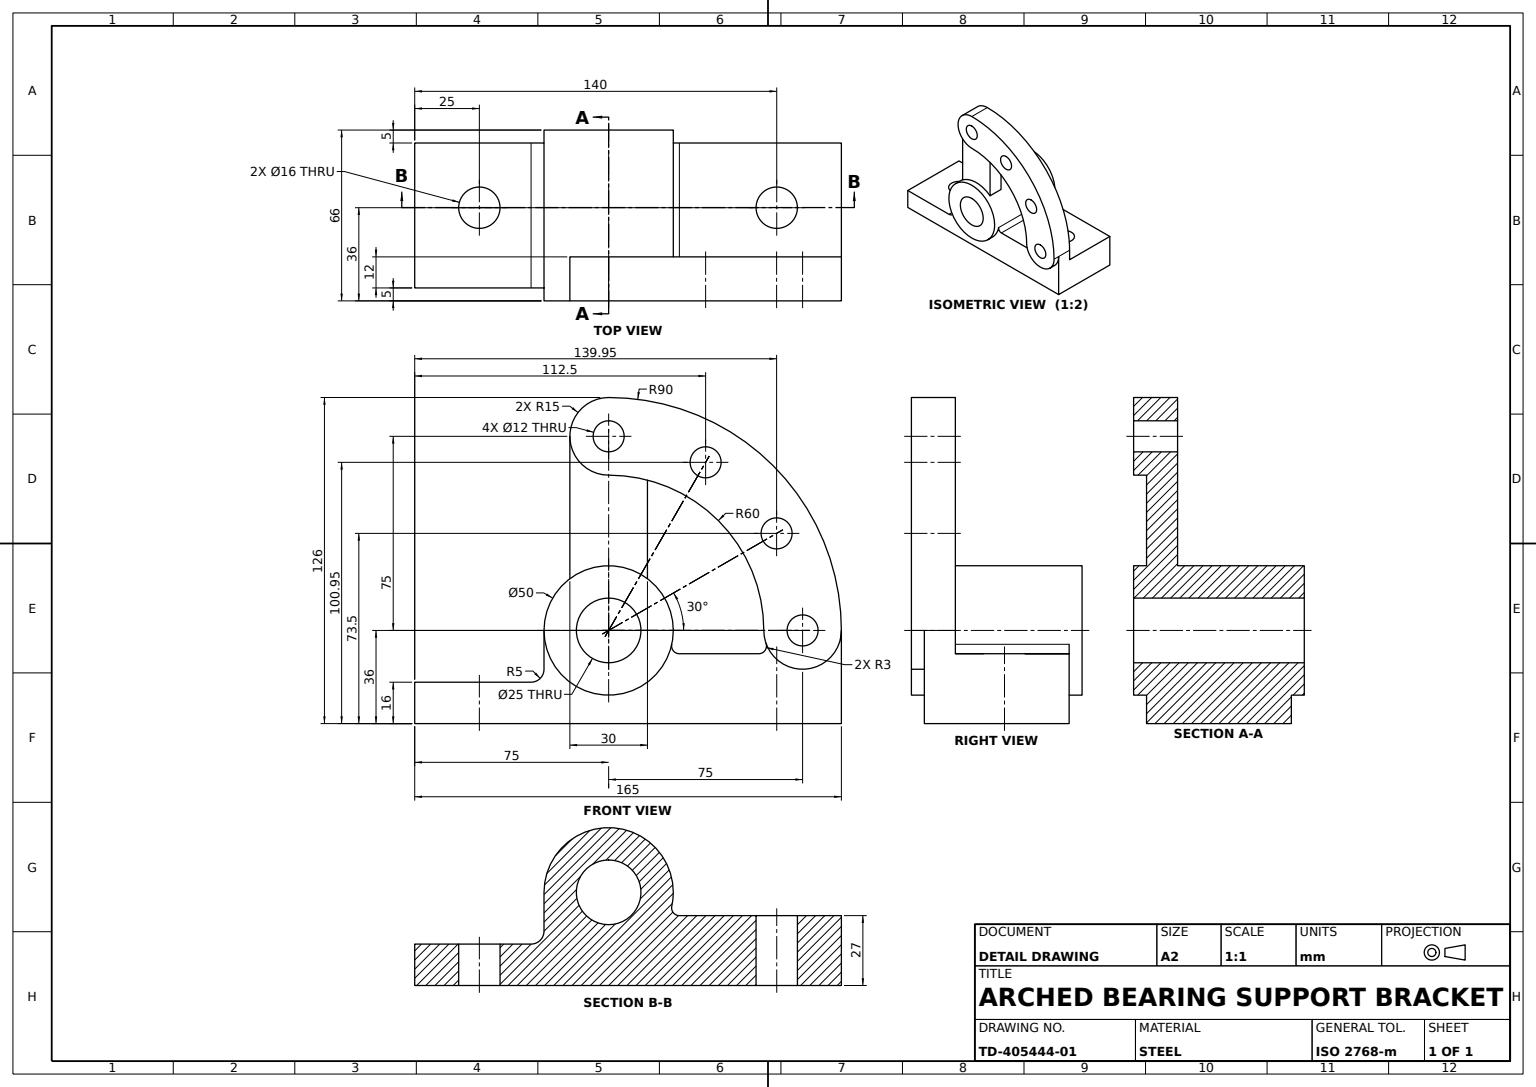
ISO-10303-21;
HEADER;
FILE_DESCRIPTION((''),'2;1');
FILE_NAME('','',(''),(''),'','','');
FILE_SCHEMA(('AUTOMOTIVE_DESIGN'));
ENDSEC;
DATA;
#1=APPLICATION_CONTEXT('');
#2=PRODUCT_CONTEXT('',#1,'mechanical');
#3=PRODUCT('','','',(#2));
#4=PRODUCT_DEFINITION_FORMATION('','',#3);
#5=PRODUCT_DEFINITION_CONTEXT('',#1,'design');
#6=PRODUCT_DEFINITION('','',#4,#5);
#7=PRODUCT_DEFINITION_SHAPE('','',#6);
#8=(LENGTH_UNIT()NAMED_UNIT(*)SI_UNIT(.MILLI.,.METRE.));
#9=(NAMED_UNIT(*)PLANE_ANGLE_UNIT()SI_UNIT($,.RADIAN.));
#10=(NAMED_UNIT(*)SI_UNIT($,.STERADIAN.)SOLID_ANGLE_UNIT());
#11=UNCERTAINTY_MEASURE_WITH_UNIT(LENGTH_MEASURE(0.005),#8,'distance_accuracy_value','');
#12=(GEOMETRIC_REPRESENTATION_CONTEXT(3)GLOBAL_UNCERTAINTY_ASSIGNED_CONTEXT((#11))GLOBAL_UNIT_ASSIGNED_CONTEXT((#8,#9,#10))REPRESENTATION_CONTEXT('',''));
#13=CARTESIAN_POINT('',(-11.,-50.,16.));
#14=VERTEX_POINT('',#13);
#15=CARTESIAN_POINT('',(-3.,-50.,16.));
#16=DIRECTION('',(0.,0.,-1.));
#17=DIRECTION('',(-1.,0.,0.));
#18=AXIS2_PLACEMENT_3D('',#15,#16,#17);
#19=CIRCLE('',#18,8.);
#20=EDGE_CURVE('',#14,#14,#19,.T.);
#21=ORIENTED_EDGE('',*,*,#20,.F.);
#22=EDGE_LOOP('',(#21));
#23=FACE_BOUND('',#22,.T.);
#24=CARTESIAN_POINT('',(5.,-50.,0.));
#25=VERTEX_POINT('',#24);
#26=CARTESIAN_POINT('',(-3.,-50.,0.));
#27=DIRECTION('',(0.,0.,1.));
#28=DIRECTION('',(1.,0.,0.));
#29=AXIS2_PLACEMENT_3D('',#26,#27,#28);
#30=CIRCLE('',#29,8.);
#31=EDGE_CURVE('',#25,#25,#30,.T.);
#32=ORIENTED_EDGE('',*,*,#31,.F.);
#33=EDGE_LOOP('',(#32));
#34=FACE_BOUND('',#33,.T.);
#35=CYLINDRICAL_SURFACE('',#29,8.);
#36=ADVANCED_FACE('',(#23,#34),#35,.F.);
#37=CARTESIAN_POINT('',(28.,-75.,16.));
#38=VERTEX_POINT('',#37);
#39=CARTESIAN_POINT('',(28.,-75.,0.));
#40=VERTEX_POINT('',#39);
#41=VECTOR('',#16,1000.);
#42=LINE('',#37,#41);
#43=EDGE_CURVE('',#38,#40,#42,.T.);
#44=ORIENTED_EDGE('',*,*,#43,.F.);
#45=CARTESIAN_POINT('',(-28.,-75.,16.));
#46=VERTEX_POINT('',#45);
#47=VECTOR('',#17,1000.);
#48=LINE('',#37,#47);
#49=EDGE_CURVE('',#38,#46,#48,.T.);
#50=ORIENTED_EDGE('',*,*,#49,.T.);
#51=CARTESIAN_POINT('',(-28.,-75.,0.));
#52=VERTEX_POINT('',#51);
#53=LINE('',#45,#41);
#54=EDGE_CURVE('',#46,#52,#53,.T.);
#55=ORIENTED_EDGE('',*,*,#54,.T.);
#56=LINE('',#39,#47);
#57=EDGE_CURVE('',#40,#52,#56,.T.);
#58=ORIENTED_EDGE('',*,*,#57,.F.);
#59=EDGE_LOOP('',(#44,#50,#55,#58));
#60=FACE_BOUND('',#59,.T.);
#61=DIRECTION('',(0.,1.,0.));
#62=AXIS2_PLACEMENT_3D('',#37,#61,#27);
#63=PLANE('',#62);
#64=ADVANCED_FACE('',(#60),#63,.F.);
#65=CARTESIAN_POINT('',(16.,-15.,56.));
#66=VERTEX_POINT('',#65);
#67=CARTESIAN_POINT('',(28.,-15.,56.));
#68=VERTEX_POINT('',#67);
#69=CARTESIAN_POINT('',(33.,-15.,56.));
#70=LINE('',#69,#47);
#71=EDGE_CURVE('',#66,#68,#70,.F.);
#72=ORIENTED_EDGE('',*,*,#71,.T.);
#73=CARTESIAN_POINT('',(28.,-15.,111.));
#74=VERTEX_POINT('',#73);
#75=LINE('',#73,#41);
#76=EDGE_CURVE('',#74,#68,#75,.T.);
#77=ORIENTED_EDGE('',*,*,#76,.F.);
#78=CARTESIAN_POINT('',(16.,-15.,111.));
#79=VERTEX_POINT('',#78);
#80=LINE('',#73,#47);
#81=EDGE_CURVE('',#74,#79,#80,.T.);
#82=ORIENTED_EDGE('',*,*,#81,.T.);
#83=LINE('',#78,#41);
#84=EDGE_CURVE('',#79,#66,#83,.T.);
#85=ORIENTED_EDGE('',*,*,#84,.T.);
#86=EDGE_LOOP('',(#72,#77,#82,#85));
#87=FACE_BOUND('',#86,.T.);
#88=AXIS2_PLACEMENT_3D('',#73,#61,#27);
#89=PLANE('',#88);
#90=ADVANCED_FACE('',(#87),#89,.F.);
#91=ORIENTED_EDGE('',*,*,#20,.T.);
#92=EDGE_LOOP('',(#91));
#93=FACE_BOUND('',#92,.T.);
#94=ORIENTED_EDGE('',*,*,#49,.F.);
#95=CARTESIAN_POINT('',(28.,-30.,16.));
#96=VERTEX_POINT('',#95);
#97=CARTESIAN_POINT('',(28.,-15.,16.));
#98=DIRECTION('',(0.,-1.,0.));
#99=VECTOR('',#98,1000.);
#100=LINE('',#97,#99);
#101=EDGE_CURVE('',#96,#38,#100,.T.);
#102=ORIENTED_EDGE('',*,*,#101,.F.);
#103=CARTESIAN_POINT('',(-28.,-30.,16.));
#104=VERTEX_POINT('',#103);
#105=LINE('',#103,#47);
#106=EDGE_CURVE('',#96,#104,#105,.T.);
#107=ORIENTED_EDGE('',*,*,#106,.T.);
#108=CARTESIAN_POINT('',(-28.,-15.,16.));
#109=LINE('',#108,#99);
#110=EDGE_CURVE('',#104,#46,#109,.T.);
#111=ORIENTED_EDGE('',*,*,#110,.T.);
#112=EDGE_LOOP('',(#94,#102,#107,#111));
#113=FACE_BOUND('',#112,.T.);
#114=AXIS2_PLACEMENT_3D('',#97,#16,#17);
#115=PLANE('',#114);
#116=ADVANCED_FACE('',(#93,#113),#115,.F.);
#117=CARTESIAN_POINT('',(-33.,0.,23.5));
#118=VERTEX_POINT('',#117);
#119=CARTESIAN_POINT('',(-33.,0.,36.));
#120=AXIS2_PLACEMENT_3D('',#119,#28,#16);
#121=CIRCLE('',#120,12.5);
#122=EDGE_CURVE('',#118,#118,#121,.T.);
#123=ORIENTED_EDGE('',*,*,#122,.F.);
#124=EDGE_LOOP('',(#123));
#125=FACE_BOUND('',#124,.T.);
#126=CARTESIAN_POINT('',(33.,0.,48.5));
#127=VERTEX_POINT('',#126);
#128=CARTESIAN_POINT('',(33.,0.,36.));
#129=AXIS2_PLACEMENT_3D('',#128,#17,#27);
#130=CIRCLE('',#129,12.5);
#131=EDGE_CURVE('',#127,#127,#130,.T.);
#132=ORIENTED_EDGE('',*,*,#131,.F.);
#133=EDGE_LOOP('',(#132));
#134=FACE_BOUND('',#133,.T.);
#135=CYLINDRICAL_SURFACE('',#129,12.5);
#136=ADVANCED_FACE('',(#125,#134),#135,.F.);
#137=ORIENTED_EDGE('',*,*,#122,.T.);
#138=EDGE_LOOP('',(#137));
#139=FACE_BOUND('',#138,.T.);
#140=CARTESIAN_POINT('',(-33.,25.,36.));
#141=VERTEX_POINT('',#140);
#142=AXIS2_PLACEMENT_3D('',#119,#28,#61);
#143=CIRCLE('',#142,25.);
#144=EDGE_CURVE('',#141,#141,#143,.T.);
#145=ORIENTED_EDGE('',*,*,#144,.F.);
#146=EDGE_LOOP('',(#145));
#147=FACE_BOUND('',#146,.T.);
#148=PLANE('',#120);
#149=ADVANCED_FACE('',(#139,#147),#148,.F.);
#150=CARTESIAN_POINT('',(28.,58.029437,27.));
#151=VERTEX_POINT('',#150);
#152=CARTESIAN_POINT('',(16.,58.029437,27.));
#153=VERTEX_POINT('',#152);
#154=VECTOR('',#28,1000.);
#155=LINE('',#152,#154);
#156=EDGE_CURVE('',#151,#153,#155,.F.);
#157=ORIENTED_EDGE('',*,*,#156,.F.);
#158=CARTESIAN_POINT('',(28.,60.857864,31.));
#159=VERTEX_POINT('',#158);
#160=CARTESIAN_POINT('',(28.,58.029437,30.));
#161=AXIS2_PLACEMENT_3D('',#160,#28,#16);
#162=CIRCLE('',#161,3.);
#163=EDGE_CURVE('',#159,#151,#162,.F.);
#164=ORIENTED_EDGE('',*,*,#163,.F.);
#165=CARTESIAN_POINT('',(16.,60.857864,31.));
#166=VERTEX_POINT('',#165);
#167=CARTESIAN_POINT('',(33.,60.857864,31.));
#168=LINE('',#167,#47);
#169=EDGE_CURVE('',#166,#159,#168,.F.);
#170=ORIENTED_EDGE('',*,*,#169,.F.);
#171=CARTESIAN_POINT('',(16.,58.029437,30.));
#172=AXIS2_PLACEMENT_3D('',#171,#28,#16);
#173=CIRCLE('',#172,3.);
#174=EDGE_CURVE('',#153,#166,#173,.T.);
#175=ORIENTED_EDGE('',*,*,#174,.F.);
#176=EDGE_LOOP('',(#157,#164,#170,#175));
#177=FACE_BOUND('',#176,.T.);
#178=CARTESIAN_POINT('',(33.,58.029437,30.));
#179=AXIS2_PLACEMENT_3D('',#178,#17,#27);
#180=CYLINDRICAL_SURFACE('',#179,3.);
#181=ADVANCED_FACE('',(#177),#180,.F.);
#182=CARTESIAN_POINT('',(28.,15.,56.));
#183=VERTEX_POINT('',#182);
#184=CARTESIAN_POINT('',(16.,15.,56.));
#185=VERTEX_POINT('',#184);
#186=CARTESIAN_POINT('',(33.,15.,56.));
#187=LINE('',#186,#47);
#188=EDGE_CURVE('',#183,#185,#187,.T.);
#189=ORIENTED_EDGE('',*,*,#188,.F.);
#190=CARTESIAN_POINT('',(28.,0.,36.));
#191=AXIS2_PLACEMENT_3D('',#190,#28,#16);
#192=CIRCLE('',#191,25.);
#193=EDGE_CURVE('',#183,#68,#192,.T.);
#194=ORIENTED_EDGE('',*,*,#193,.T.);
#195=ORIENTED_EDGE('',*,*,#71,.F.);
#196=CARTESIAN_POINT('',(16.,0.,36.));
#197=AXIS2_PLACEMENT_3D('',#196,#28,#16);
#198=CIRCLE('',#197,25.);
#199=EDGE_CURVE('',#185,#66,#198,.T.);
#200=ORIENTED_EDGE('',*,*,#199,.F.);
#201=EDGE_LOOP('',(#189,#194,#195,#200));
#202=FACE_BOUND('',#201,.T.);
#203=CARTESIAN_POINT('',(33.,25.,36.));
#204=VERTEX_POINT('',#203);
#205=AXIS2_PLACEMENT_3D('',#128,#28,#61);
#206=CIRCLE('',#205,25.);
#207=EDGE_CURVE('',#204,#204,#206,.T.);
#208=ORIENTED_EDGE('',*,*,#207,.F.);
#209=EDGE_LOOP('',(#208));
#210=FACE_BOUND('',#209,.T.);
#211=CARTESIAN_POINT('',(28.,24.419276,30.642857));
#212=VERTEX_POINT('',#211);
#213=CARTESIAN_POINT('',(-28.,24.419276,30.642857));
#214=VERTEX_POINT('',#213);
#215=CARTESIAN_POINT('',(33.,24.419276,30.642857));
#216=LINE('',#215,#47);
#217=EDGE_CURVE('',#212,#214,#216,.T.);
#218=ORIENTED_EDGE('',*,*,#217,.T.);
#219=CARTESIAN_POINT('',(-28.,-25.,36.));
#220=VERTEX_POINT('',#219);
#221=CARTESIAN_POINT('',(-28.,0.,36.));
#222=AXIS2_PLACEMENT_3D('',#221,#28,#16);
#223=CIRCLE('',#222,25.);
#224=EDGE_CURVE('',#214,#220,#223,.F.);
#225=ORIENTED_EDGE('',*,*,#224,.T.);
#226=CARTESIAN_POINT('',(28.,-25.,36.));
#227=VERTEX_POINT('',#226);
#228=LINE('',#226,#47);
#229=EDGE_CURVE('',#227,#220,#228,.T.);
#230=ORIENTED_EDGE('',*,*,#229,.F.);
#231=EDGE_CURVE('',#212,#227,#192,.F.);
#232=ORIENTED_EDGE('',*,*,#231,.F.);
#233=EDGE_LOOP('',(#218,#225,#230,#232));
#234=FACE_BOUND('',#233,.T.);
#235=ORIENTED_EDGE('',*,*,#144,.T.);
#236=EDGE_LOOP('',(#235));
#237=FACE_BOUND('',#236,.T.);
#238=CYLINDRICAL_SURFACE('',#129,25.);
#239=ADVANCED_FACE('',(#202,#210,#234,#237),#238,.T.);
#240=CARTESIAN_POINT('',(16.,0.,105.));
#241=VERTEX_POINT('',#240);
#242=CARTESIAN_POINT('',(16.,0.,111.));
#243=AXIS2_PLACEMENT_3D('',#242,#28,#16);
#244=CIRCLE('',#243,6.);
#245=EDGE_CURVE('',#241,#241,#244,.T.);
#246=ORIENTED_EDGE('',*,*,#245,.T.);
#247=EDGE_LOOP('',(#246));
#248=FACE_BOUND('',#247,.T.);
#249=CARTESIAN_POINT('',(16.,64.951905,67.5));
#250=VERTEX_POINT('',#249);
#251=CARTESIAN_POINT('',(16.,64.951905,73.5));
#252=AXIS2_PLACEMENT_3D('',#251,#28,#16);
#253=CIRCLE('',#252,6.);
#254=EDGE_CURVE('',#250,#250,#253,.T.);
#255=ORIENTED_EDGE('',*,*,#254,.T.);
#256=EDGE_LOOP('',(#255));
#257=FACE_BOUND('',#256,.T.);
#258=CARTESIAN_POINT('',(16.,75.,30.));
#259=VERTEX_POINT('',#258);
#260=CARTESIAN_POINT('',(16.,75.,36.));
#261=AXIS2_PLACEMENT_3D('',#260,#28,#16);
#262=CIRCLE('',#261,6.);
#263=EDGE_CURVE('',#259,#259,#262,.T.);
#264=ORIENTED_EDGE('',*,*,#263,.T.);
#265=EDGE_LOOP('',(#264));
#266=FACE_BOUND('',#265,.T.);
#267=CARTESIAN_POINT('',(16.,37.5,94.951905));
#268=VERTEX_POINT('',#267);
#269=CARTESIAN_POINT('',(16.,37.5,100.951905));
#270=AXIS2_PLACEMENT_3D('',#269,#28,#16);
#271=CIRCLE('',#270,6.);
#272=EDGE_CURVE('',#268,#268,#271,.T.);
#273=ORIENTED_EDGE('',*,*,#272,.T.);
#274=EDGE_LOOP('',(#273));
#275=FACE_BOUND('',#274,.T.);
#276=CARTESIAN_POINT('',(16.,60.,36.));
#277=VERTEX_POINT('',#276);
#278=AXIS2_PLACEMENT_3D('',#260,#28,#61);
#279=CIRCLE('',#278,15.);
#280=EDGE_CURVE('',#277,#166,#279,.T.);
#281=ORIENTED_EDGE('',*,*,#280,.F.);
#282=CARTESIAN_POINT('',(16.,15.,94.09475));
#283=VERTEX_POINT('',#282);
#284=AXIS2_PLACEMENT_3D('',#196,#17,#61);
#285=CIRCLE('',#284,60.);
#286=EDGE_CURVE('',#283,#277,#285,.T.);
#287=ORIENTED_EDGE('',*,*,#286,.F.);
#288=CARTESIAN_POINT('',(16.,15.,36.));
#289=VECTOR('',#27,1000.);
#290=LINE('',#288,#289);
#291=EDGE_CURVE('',#185,#283,#290,.T.);
#292=ORIENTED_EDGE('',*,*,#291,.F.);
#293=ORIENTED_EDGE('',*,*,#199,.T.);
#294=ORIENTED_EDGE('',*,*,#84,.F.);
#295=CARTESIAN_POINT('',(16.,0.,126.));
#296=VERTEX_POINT('',#295);
#297=AXIS2_PLACEMENT_3D('',#242,#28,#61);
#298=CIRCLE('',#297,15.);
#299=EDGE_CURVE('',#296,#79,#298,.T.);
#300=ORIENTED_EDGE('',*,*,#299,.F.);
#301=CARTESIAN_POINT('',(16.,90.,36.));
#302=VERTEX_POINT('',#301);
#303=CARTESIAN_POINT('',(16.,2.954652,126.));
#304=CARTESIAN_POINT('',(16.,8.831394,125.712442));
#305=CARTESIAN_POINT('',(16.,20.505808,123.979142));
#306=CARTESIAN_POINT('',(16.,34.662692,119.685644));
#307=CARTESIAN_POINT('',(16.,50.323854,111.31453));
#308=CARTESIAN_POINT('',(16.,64.049819,100.049825));
#309=CARTESIAN_POINT('',(16.,75.314532,86.323832));
#310=CARTESIAN_POINT('',(16.,83.685644,70.662772));
#311=CARTESIAN_POINT('',(16.,87.979142,56.505573));
#312=CARTESIAN_POINT('',(16.,89.712442,44.831801));
#313=CARTESIAN_POINT('',(16.,90.,38.954832));
#314=B_SPLINE_CURVE_WITH_KNOTS('',3,(#295,#303,#304,#305,#306,#307,#308,#309,#310,#311,#312,#313,#301),.UNSPECIFIED.,.F.,.F.,(4,1,1,1,1,1,1,1,1,1,4),(0.,0.0625,0.125,0.25,0.375,0.5,0.625,0.75,0.875,0.9375,1.),.UNSPECIFIED.);
#315=EDGE_CURVE('',#302,#296,#314,.F.);
#316=ORIENTED_EDGE('',*,*,#315,.F.);
#317=CARTESIAN_POINT('',(16.,90.,27.));
#318=VERTEX_POINT('',#317);
#319=CARTESIAN_POINT('',(16.,90.,30.));
#320=CARTESIAN_POINT('',(16.,90.,33.));
#321=B_SPLINE_CURVE_WITH_KNOTS('',3,(#317,#319,#320,#301),.UNSPECIFIED.,.F.,.F.,(4,4),(0.59699429,0.993877832),.UNSPECIFIED.);
#322=EDGE_CURVE('',#302,#318,#321,.F.);
#323=ORIENTED_EDGE('',*,*,#322,.T.);
#324=LINE('',#317,#99);
#325=EDGE_CURVE('',#318,#153,#324,.T.);
#326=ORIENTED_EDGE('',*,*,#325,.T.);
#327=ORIENTED_EDGE('',*,*,#174,.T.);
#328=EDGE_LOOP('',(#281,#287,#292,#293,#294,#300,#316,#323,#326,#327));
#329=FACE_BOUND('',#328,.T.);
#330=CARTESIAN_POINT('',(16.,0.,0.));
#331=AXIS2_PLACEMENT_3D('',#330,#28,#16);
#332=PLANE('',#331);
#333=ADVANCED_FACE('',(#248,#257,#266,#275,#329),#332,.F.);
#334=CARTESIAN_POINT('',(-3.,73.,27.));
#335=VERTEX_POINT('',#334);
#336=CARTESIAN_POINT('',(-3.,65.,27.));
#337=AXIS2_PLACEMENT_3D('',#336,#16,#61);
#338=CIRCLE('',#337,8.);
#339=EDGE_CURVE('',#335,#335,#338,.T.);
#340=ORIENTED_EDGE('',*,*,#339,.T.);
#341=EDGE_LOOP('',(#340));
#342=FACE_BOUND('',#341,.T.);
#343=CARTESIAN_POINT('',(-28.,90.,27.));
#344=VERTEX_POINT('',#343);
#345=CARTESIAN_POINT('',(28.,90.,27.));
#346=LINE('',#345,#47);
#347=EDGE_CURVE('',#318,#344,#346,.T.);
#348=ORIENTED_EDGE('',*,*,#347,.T.);
#349=CARTESIAN_POINT('',(-28.,27.349589,27.));
#350=VERTEX_POINT('',#349);
#351=LINE('',#343,#99);
#352=EDGE_CURVE('',#344,#350,#351,.T.);
#353=ORIENTED_EDGE('',*,*,#352,.T.);
#354=CARTESIAN_POINT('',(28.,27.349589,27.));
#355=VERTEX_POINT('',#354);
#356=LINE('',#354,#154);
#357=EDGE_CURVE('',#350,#355,#356,.T.);
#358=ORIENTED_EDGE('',*,*,#357,.T.);
#359=LINE('',#345,#99);
#360=EDGE_CURVE('',#151,#355,#359,.T.);
#361=ORIENTED_EDGE('',*,*,#360,.F.);
#362=ORIENTED_EDGE('',*,*,#156,.T.);
#363=ORIENTED_EDGE('',*,*,#325,.F.);
#364=EDGE_LOOP('',(#348,#353,#358,#361,#362,#363));
#365=FACE_BOUND('',#364,.T.);
#366=AXIS2_PLACEMENT_3D('',#345,#16,#61);
#367=PLANE('',#366);
#368=ADVANCED_FACE('',(#342,#365),#367,.F.);
#369=CARTESIAN_POINT('',(33.,64.951905,79.5));
#370=VERTEX_POINT('',#369);
#371=CARTESIAN_POINT('',(33.,64.951905,73.5));
#372=AXIS2_PLACEMENT_3D('',#371,#17,#27);
#373=CIRCLE('',#372,6.);
#374=EDGE_CURVE('',#370,#370,#373,.T.);
#375=ORIENTED_EDGE('',*,*,#374,.F.);
#376=EDGE_LOOP('',(#375));
#377=FACE_BOUND('',#376,.T.);
#378=ORIENTED_EDGE('',*,*,#254,.F.);
#379=EDGE_LOOP('',(#378));
#380=FACE_BOUND('',#379,.T.);
#381=CYLINDRICAL_SURFACE('',#372,6.);
#382=ADVANCED_FACE('',(#377,#380),#381,.F.);
#383=CARTESIAN_POINT('',(28.,90.,36.));
#384=VERTEX_POINT('',#383);
#385=CARTESIAN_POINT('',(28.,75.,36.));
#386=AXIS2_PLACEMENT_3D('',#385,#28,#16);
#387=CIRCLE('',#386,15.);
#388=EDGE_CURVE('',#384,#159,#387,.F.);
#389=ORIENTED_EDGE('',*,*,#388,.F.);
#390=CARTESIAN_POINT('',(33.,90.,36.));
#391=VERTEX_POINT('',#390);
#392=LINE('',#390,#47);
#393=EDGE_CURVE('',#391,#384,#392,.T.);
#394=ORIENTED_EDGE('',*,*,#393,.F.);
#395=CARTESIAN_POINT('',(33.,60.,36.));
#396=VERTEX_POINT('',#395);
#397=CARTESIAN_POINT('',(33.,75.,36.));
#398=AXIS2_PLACEMENT_3D('',#397,#28,#61);
#399=CIRCLE('',#398,15.);
#400=EDGE_CURVE('',#396,#391,#399,.T.);
#401=ORIENTED_EDGE('',*,*,#400,.F.);
#402=LINE('',#395,#47);
#403=EDGE_CURVE('',#396,#277,#402,.T.);
#404=ORIENTED_EDGE('',*,*,#403,.T.);
#405=ORIENTED_EDGE('',*,*,#280,.T.);
#406=ORIENTED_EDGE('',*,*,#169,.T.);
#407=EDGE_LOOP('',(#389,#394,#401,#404,#405,#406));
#408=FACE_BOUND('',#407,.T.);
#409=AXIS2_PLACEMENT_3D('',#397,#17,#27);
#410=CYLINDRICAL_SURFACE('',#409,15.);
#411=ADVANCED_FACE('',(#408),#410,.T.);
#412=CARTESIAN_POINT('',(28.,15.,94.09475));
#413=VERTEX_POINT('',#412);
#414=CARTESIAN_POINT('',(28.,15.,36.));
#415=LINE('',#414,#289);
#416=EDGE_CURVE('',#183,#413,#415,.T.);
#417=ORIENTED_EDGE('',*,*,#416,.T.);
#418=CARTESIAN_POINT('',(28.,0.,96.));
#419=VERTEX_POINT('',#418);
#420=CIRCLE('',#191,60.);
#421=EDGE_CURVE('',#413,#419,#420,.T.);
#422=ORIENTED_EDGE('',*,*,#421,.T.);
#423=CARTESIAN_POINT('',(28.,0.,111.));
#424=AXIS2_PLACEMENT_3D('',#423,#28,#16);
#425=CIRCLE('',#424,15.);
#426=EDGE_CURVE('',#419,#74,#425,.F.);
#427=ORIENTED_EDGE('',*,*,#426,.T.);
#428=ORIENTED_EDGE('',*,*,#76,.T.);
#429=ORIENTED_EDGE('',*,*,#193,.F.);
#430=EDGE_LOOP('',(#417,#422,#427,#428,#429));
#431=FACE_BOUND('',#430,.T.);
#432=CARTESIAN_POINT('',(28.,0.,0.));
#433=AXIS2_PLACEMENT_3D('',#432,#28,#16);
#434=PLANE('',#433);
#435=ADVANCED_FACE('',(#431),#434,.T.);
#436=VERTEX_POINT('',#345);
#437=CARTESIAN_POINT('',(28.,90.,33.));
#438=CARTESIAN_POINT('',(28.,90.,30.));
#439=B_SPLINE_CURVE_WITH_KNOTS('',3,(#383,#437,#438,#345),.UNSPECIFIED.,.F.,.F.,(4,4),(0.006122168,0.40300571),.UNSPECIFIED.);
#440=EDGE_CURVE('',#436,#384,#439,.F.);
#441=ORIENTED_EDGE('',*,*,#440,.T.);
#442=ORIENTED_EDGE('',*,*,#388,.T.);
#443=ORIENTED_EDGE('',*,*,#163,.T.);
#444=ORIENTED_EDGE('',*,*,#360,.T.);
#445=CARTESIAN_POINT('',(28.,27.349589,30.));
#446=AXIS2_PLACEMENT_3D('',#445,#28,#16);
#447=CIRCLE('',#446,3.);
#448=EDGE_CURVE('',#355,#212,#447,.F.);
#449=ORIENTED_EDGE('',*,*,#448,.T.);
#450=ORIENTED_EDGE('',*,*,#231,.T.);
#451=CARTESIAN_POINT('',(28.,-25.,21.));
#452=VERTEX_POINT('',#451);
#453=LINE('',#226,#41);
#454=EDGE_CURVE('',#227,#452,#453,.T.);
#455=ORIENTED_EDGE('',*,*,#454,.T.);
#456=CARTESIAN_POINT('',(28.,-30.,21.));
#457=AXIS2_PLACEMENT_3D('',#456,#28,#16);
#458=CIRCLE('',#457,5.);
#459=EDGE_CURVE('',#452,#96,#458,.F.);
#460=ORIENTED_EDGE('',*,*,#459,.T.);
#461=ORIENTED_EDGE('',*,*,#101,.T.);
#462=ORIENTED_EDGE('',*,*,#43,.T.);
#463=CARTESIAN_POINT('',(28.,90.,0.));
#464=VERTEX_POINT('',#463);
#465=VECTOR('',#61,1000.);
#466=LINE('',#39,#465);
#467=EDGE_CURVE('',#40,#464,#466,.T.);
#468=ORIENTED_EDGE('',*,*,#467,.T.);
#469=LINE('',#463,#289);
#470=EDGE_CURVE('',#464,#436,#469,.T.);
#471=ORIENTED_EDGE('',*,*,#470,.T.);
#472=EDGE_LOOP('',(#441,#442,#443,#444,#449,#450,#455,#460,#461,#462,#468,#471));
#473=FACE_BOUND('',#472,.T.);
#474=ADVANCED_FACE('',(#473),#434,.T.);
#475=ORIENTED_EDGE('',*,*,#291,.T.);
#476=CARTESIAN_POINT('',(33.,15.,94.09475));
#477=LINE('',#476,#47);
#478=EDGE_CURVE('',#413,#283,#477,.T.);
#479=ORIENTED_EDGE('',*,*,#478,.F.);
#480=ORIENTED_EDGE('',*,*,#416,.F.);
#481=ORIENTED_EDGE('',*,*,#188,.T.);
#482=EDGE_LOOP('',(#475,#479,#480,#481));
#483=FACE_BOUND('',#482,.T.);
#484=AXIS2_PLACEMENT_3D('',#414,#98,#16);
#485=PLANE('',#484);
#486=ADVANCED_FACE('',(#483),#485,.F.);
#487=CARTESIAN_POINT('',(33.,0.,126.));
#488=VERTEX_POINT('',#487);
#489=CIRCLE('',#205,90.);
#490=EDGE_CURVE('',#391,#488,#489,.T.);
#491=ORIENTED_EDGE('',*,*,#490,.T.);
#492=CARTESIAN_POINT('',(33.,0.,96.));
#493=VERTEX_POINT('',#492);
#494=CARTESIAN_POINT('',(33.,0.,111.));
#495=AXIS2_PLACEMENT_3D('',#494,#28,#61);
#496=CIRCLE('',#495,15.);
#497=EDGE_CURVE('',#488,#493,#496,.T.);
#498=ORIENTED_EDGE('',*,*,#497,.T.);
#499=AXIS2_PLACEMENT_3D('',#128,#17,#61);
#500=CIRCLE('',#499,60.);
#501=EDGE_CURVE('',#493,#396,#500,.T.);
#502=ORIENTED_EDGE('',*,*,#501,.T.);
#503=ORIENTED_EDGE('',*,*,#400,.T.);
#504=EDGE_LOOP('',(#491,#498,#502,#503));
#505=FACE_BOUND('',#504,.T.);
#506=CARTESIAN_POINT('',(33.,37.5,106.951905));
#507=VERTEX_POINT('',#506);
#508=CARTESIAN_POINT('',(33.,37.5,100.951905));
#509=AXIS2_PLACEMENT_3D('',#508,#17,#27);
#510=CIRCLE('',#509,6.);
#511=EDGE_CURVE('',#507,#507,#510,.T.);
#512=ORIENTED_EDGE('',*,*,#511,.T.);
#513=EDGE_LOOP('',(#512));
#514=FACE_BOUND('',#513,.T.);
#515=CARTESIAN_POINT('',(33.,75.,42.));
#516=VERTEX_POINT('',#515);
#517=CIRCLE('',#409,6.);
#518=EDGE_CURVE('',#516,#516,#517,.T.);
#519=ORIENTED_EDGE('',*,*,#518,.T.);
#520=EDGE_LOOP('',(#519));
#521=FACE_BOUND('',#520,.T.);
#522=ORIENTED_EDGE('',*,*,#374,.T.);
#523=EDGE_LOOP('',(#522));
#524=FACE_BOUND('',#523,.T.);
#525=CARTESIAN_POINT('',(33.,0.,117.));
#526=VERTEX_POINT('',#525);
#527=AXIS2_PLACEMENT_3D('',#494,#17,#27);
#528=CIRCLE('',#527,6.);
#529=EDGE_CURVE('',#526,#526,#528,.T.);
#530=ORIENTED_EDGE('',*,*,#529,.T.);
#531=EDGE_LOOP('',(#530));
#532=FACE_BOUND('',#531,.T.);
#533=CARTESIAN_POINT('',(33.,0.,73.5));
#534=AXIS2_PLACEMENT_3D('',#533,#28,#16);
#535=PLANE('',#534);
#536=ADVANCED_FACE('',(#505,#514,#521,#524,#532),#535,.T.);
#537=CARTESIAN_POINT('',(-28.,90.,0.));
#538=VERTEX_POINT('',#537);
#539=LINE('',#51,#465);
#540=EDGE_CURVE('',#52,#538,#539,.T.);
#541=ORIENTED_EDGE('',*,*,#540,.T.);
#542=LINE('',#463,#47);
#543=EDGE_CURVE('',#464,#538,#542,.T.);
#544=ORIENTED_EDGE('',*,*,#543,.F.);
#545=ORIENTED_EDGE('',*,*,#467,.F.);
#546=ORIENTED_EDGE('',*,*,#57,.T.);
#547=EDGE_LOOP('',(#541,#544,#545,#546));
#548=FACE_BOUND('',#547,.T.);
#549=ORIENTED_EDGE('',*,*,#31,.T.);
#550=EDGE_LOOP('',(#549));
#551=FACE_BOUND('',#550,.T.);
#552=CARTESIAN_POINT('',(5.,65.,0.));
#553=VERTEX_POINT('',#552);
#554=CARTESIAN_POINT('',(-3.,65.,0.));
#555=AXIS2_PLACEMENT_3D('',#554,#27,#28);
#556=CIRCLE('',#555,8.);
#557=EDGE_CURVE('',#553,#553,#556,.T.);
#558=ORIENTED_EDGE('',*,*,#557,.T.);
#559=EDGE_LOOP('',(#558));
#560=FACE_BOUND('',#559,.T.);
#561=AXIS2_PLACEMENT_3D('',#39,#27,#28);
#562=PLANE('',#561);
#563=ADVANCED_FACE('',(#548,#551,#560),#562,.F.);
#564=ORIENTED_EDGE('',*,*,#497,.F.);
#565=LINE('',#487,#47);
#566=EDGE_CURVE('',#488,#296,#565,.T.);
#567=ORIENTED_EDGE('',*,*,#566,.T.);
#568=ORIENTED_EDGE('',*,*,#299,.T.);
#569=ORIENTED_EDGE('',*,*,#81,.F.);
#570=ORIENTED_EDGE('',*,*,#426,.F.);
#571=LINE('',#492,#47);
#572=EDGE_CURVE('',#493,#419,#571,.T.);
#573=ORIENTED_EDGE('',*,*,#572,.F.);
#574=EDGE_LOOP('',(#564,#567,#568,#569,#570,#573));
#575=FACE_BOUND('',#574,.T.);
#576=CYLINDRICAL_SURFACE('',#527,15.);
#577=ADVANCED_FACE('',(#575),#576,.T.);
#578=ORIENTED_EDGE('',*,*,#339,.F.);
#579=EDGE_LOOP('',(#578));
#580=FACE_BOUND('',#579,.T.);
#581=ORIENTED_EDGE('',*,*,#557,.F.);
#582=EDGE_LOOP('',(#581));
#583=FACE_BOUND('',#582,.T.);
#584=CYLINDRICAL_SURFACE('',#555,8.);
#585=ADVANCED_FACE('',(#580,#583),#584,.F.);
#586=ORIENTED_EDGE('',*,*,#229,.T.);
#587=CARTESIAN_POINT('',(-28.,-25.,21.));
#588=VERTEX_POINT('',#587);
#589=LINE('',#219,#41);
#590=EDGE_CURVE('',#220,#588,#589,.T.);
#591=ORIENTED_EDGE('',*,*,#590,.T.);
#592=LINE('',#451,#47);
#593=EDGE_CURVE('',#588,#452,#592,.F.);
#594=ORIENTED_EDGE('',*,*,#593,.T.);
#595=ORIENTED_EDGE('',*,*,#454,.F.);
#596=EDGE_LOOP('',(#586,#591,#594,#595));
#597=FACE_BOUND('',#596,.T.);
#598=AXIS2_PLACEMENT_3D('',#226,#61,#27);
#599=PLANE('',#598);
#600=ADVANCED_FACE('',(#597),#599,.F.);
#601=ORIENTED_EDGE('',*,*,#106,.F.);
#602=ORIENTED_EDGE('',*,*,#459,.F.);
#603=ORIENTED_EDGE('',*,*,#593,.F.);
#604=CARTESIAN_POINT('',(-28.,-30.,21.));
#605=AXIS2_PLACEMENT_3D('',#604,#28,#16);
#606=CIRCLE('',#605,5.);
#607=EDGE_CURVE('',#104,#588,#606,.T.);
#608=ORIENTED_EDGE('',*,*,#607,.F.);
#609=EDGE_LOOP('',(#601,#602,#603,#608));
#610=FACE_BOUND('',#609,.T.);
#611=CYLINDRICAL_SURFACE('',#457,5.);
#612=ADVANCED_FACE('',(#610),#611,.F.);
#613=ORIENTED_EDGE('',*,*,#245,.F.);
#614=EDGE_LOOP('',(#613));
#615=FACE_BOUND('',#614,.T.);
#616=ORIENTED_EDGE('',*,*,#529,.F.);
#617=EDGE_LOOP('',(#616));
#618=FACE_BOUND('',#617,.T.);
#619=CYLINDRICAL_SURFACE('',#527,6.);
#620=ADVANCED_FACE('',(#615,#618),#619,.F.);
#621=ORIENTED_EDGE('',*,*,#352,.F.);
#622=LINE('',#537,#289);
#623=EDGE_CURVE('',#538,#344,#622,.T.);
#624=ORIENTED_EDGE('',*,*,#623,.F.);
#625=ORIENTED_EDGE('',*,*,#540,.F.);
#626=ORIENTED_EDGE('',*,*,#54,.F.);
#627=ORIENTED_EDGE('',*,*,#110,.F.);
#628=ORIENTED_EDGE('',*,*,#607,.T.);
#629=ORIENTED_EDGE('',*,*,#590,.F.);
#630=ORIENTED_EDGE('',*,*,#224,.F.);
#631=CARTESIAN_POINT('',(-28.,27.349589,30.));
#632=AXIS2_PLACEMENT_3D('',#631,#28,#16);
#633=CIRCLE('',#632,3.);
#634=EDGE_CURVE('',#214,#350,#633,.T.);
#635=ORIENTED_EDGE('',*,*,#634,.T.);
#636=EDGE_LOOP('',(#621,#624,#625,#626,#627,#628,#629,#630,#635));
#637=FACE_BOUND('',#636,.T.);
#638=CARTESIAN_POINT('',(-28.,0.,0.));
#639=AXIS2_PLACEMENT_3D('',#638,#28,#16);
#640=PLANE('',#639);
#641=ADVANCED_FACE('',(#637),#640,.F.);
#642=ORIENTED_EDGE('',*,*,#131,.T.);
#643=EDGE_LOOP('',(#642));
#644=FACE_BOUND('',#643,.T.);
#645=ORIENTED_EDGE('',*,*,#207,.T.);
#646=EDGE_LOOP('',(#645));
#647=FACE_BOUND('',#646,.T.);
#648=AXIS2_PLACEMENT_3D('',#128,#28,#16);
#649=PLANE('',#648);
#650=ADVANCED_FACE('',(#644,#647),#649,.T.);
#651=ORIENTED_EDGE('',*,*,#511,.F.);
#652=EDGE_LOOP('',(#651));
#653=FACE_BOUND('',#652,.T.);
#654=ORIENTED_EDGE('',*,*,#272,.F.);
#655=EDGE_LOOP('',(#654));
#656=FACE_BOUND('',#655,.T.);
#657=CYLINDRICAL_SURFACE('',#509,6.);
#658=ADVANCED_FACE('',(#653,#656),#657,.F.);
#659=ORIENTED_EDGE('',*,*,#403,.F.);
#660=ORIENTED_EDGE('',*,*,#501,.F.);
#661=ORIENTED_EDGE('',*,*,#572,.T.);
#662=ORIENTED_EDGE('',*,*,#421,.F.);
#663=ORIENTED_EDGE('',*,*,#478,.T.);
#664=ORIENTED_EDGE('',*,*,#286,.T.);
#665=EDGE_LOOP('',(#659,#660,#661,#662,#663,#664));
#666=FACE_BOUND('',#665,.T.);
#667=CYLINDRICAL_SURFACE('',#129,60.);
#668=ADVANCED_FACE('',(#666),#667,.F.);
#669=ORIENTED_EDGE('',*,*,#634,.F.);
#670=ORIENTED_EDGE('',*,*,#217,.F.);
#671=ORIENTED_EDGE('',*,*,#448,.F.);
#672=ORIENTED_EDGE('',*,*,#357,.F.);
#673=EDGE_LOOP('',(#669,#670,#671,#672));
#674=FACE_BOUND('',#673,.T.);
#675=CARTESIAN_POINT('',(33.,27.349589,30.));
#676=AXIS2_PLACEMENT_3D('',#675,#17,#27);
#677=CYLINDRICAL_SURFACE('',#676,3.);
#678=ADVANCED_FACE('',(#674),#677,.F.);
#679=EDGE_CURVE('',#384,#302,#392,.T.);
#680=ORIENTED_EDGE('',*,*,#679,.F.);
#681=ORIENTED_EDGE('',*,*,#440,.F.);
#682=ORIENTED_EDGE('',*,*,#470,.F.);
#683=ORIENTED_EDGE('',*,*,#543,.T.);
#684=ORIENTED_EDGE('',*,*,#623,.T.);
#685=ORIENTED_EDGE('',*,*,#347,.F.);
#686=ORIENTED_EDGE('',*,*,#322,.F.);
#687=EDGE_LOOP('',(#680,#681,#682,#683,#684,#685,#686));
#688=FACE_BOUND('',#687,.T.);
#689=AXIS2_PLACEMENT_3D('',#463,#98,#16);
#690=PLANE('',#689);
#691=ADVANCED_FACE('',(#688),#690,.F.);
#692=ORIENTED_EDGE('',*,*,#518,.F.);
#693=EDGE_LOOP('',(#692));
#694=FACE_BOUND('',#693,.T.);
#695=ORIENTED_EDGE('',*,*,#263,.F.);
#696=EDGE_LOOP('',(#695));
#697=FACE_BOUND('',#696,.T.);
#698=CYLINDRICAL_SURFACE('',#409,6.);
#699=ADVANCED_FACE('',(#694,#697),#698,.F.);
#700=ORIENTED_EDGE('',*,*,#679,.T.);
#701=ORIENTED_EDGE('',*,*,#315,.T.);
#702=ORIENTED_EDGE('',*,*,#566,.F.);
#703=ORIENTED_EDGE('',*,*,#490,.F.);
#704=ORIENTED_EDGE('',*,*,#393,.T.);
#705=EDGE_LOOP('',(#700,#701,#702,#703,#704));
#706=FACE_BOUND('',#705,.T.);
#707=CYLINDRICAL_SURFACE('',#129,90.);
#708=ADVANCED_FACE('',(#706),#707,.T.);
#709=CLOSED_SHELL('',(#36,#64,#90,#116,#136,#149,#181,#239,#333,#368,#382,#411,#435,#474,#486,#536,#563,#577,#585,#600,#612,#620,#641,#650,#658,#668,#678,#691,#699,#708));
#710=MANIFOLD_SOLID_BREP('',#709);
#711=ADVANCED_BREP_SHAPE_REPRESENTATION('',(#710),#12);
#712=SHAPE_DEFINITION_REPRESENTATION(#7,#711);
ENDSEC;
END-ISO-10303-21;
